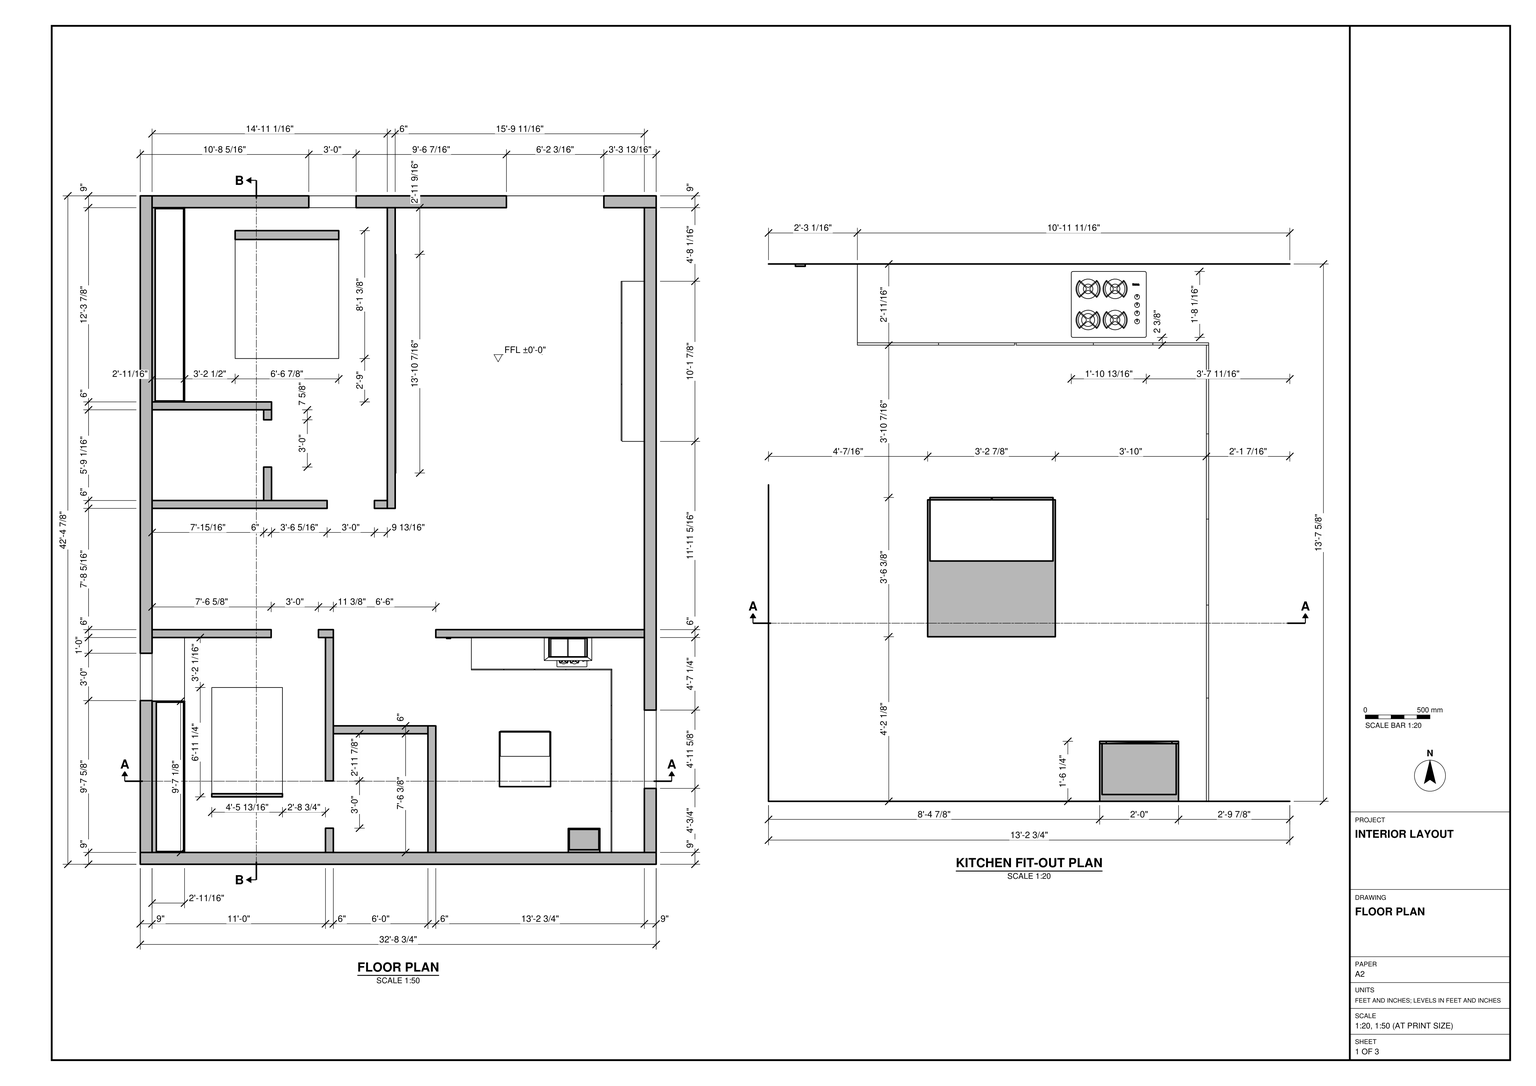
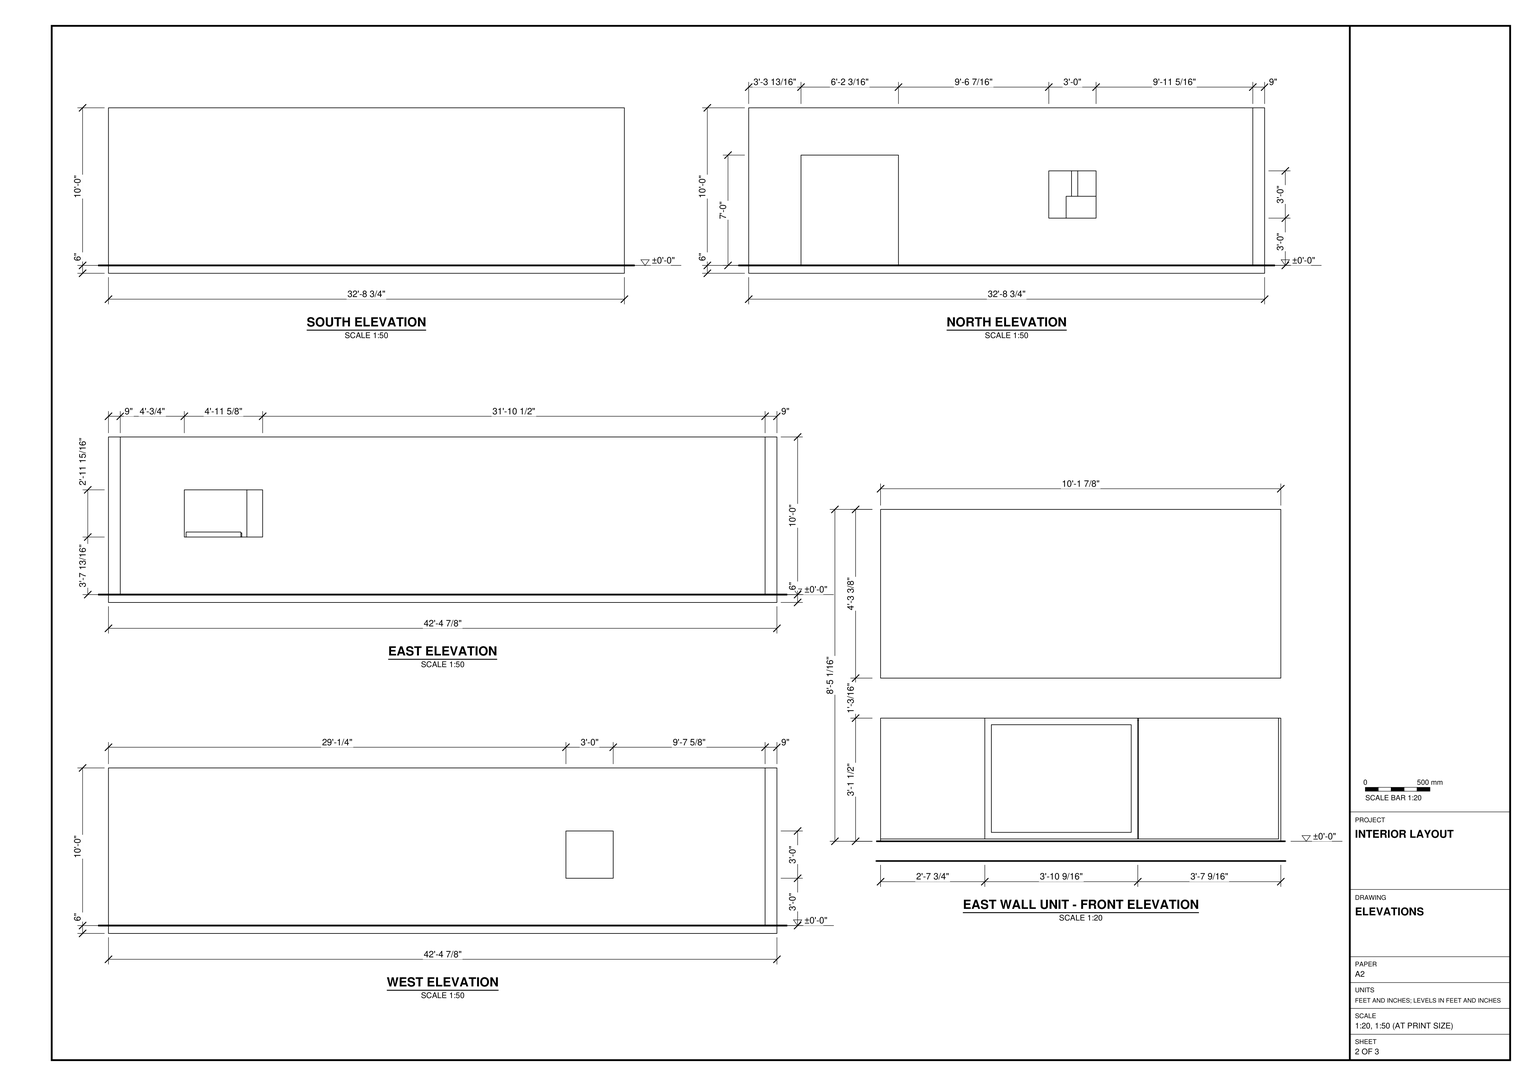
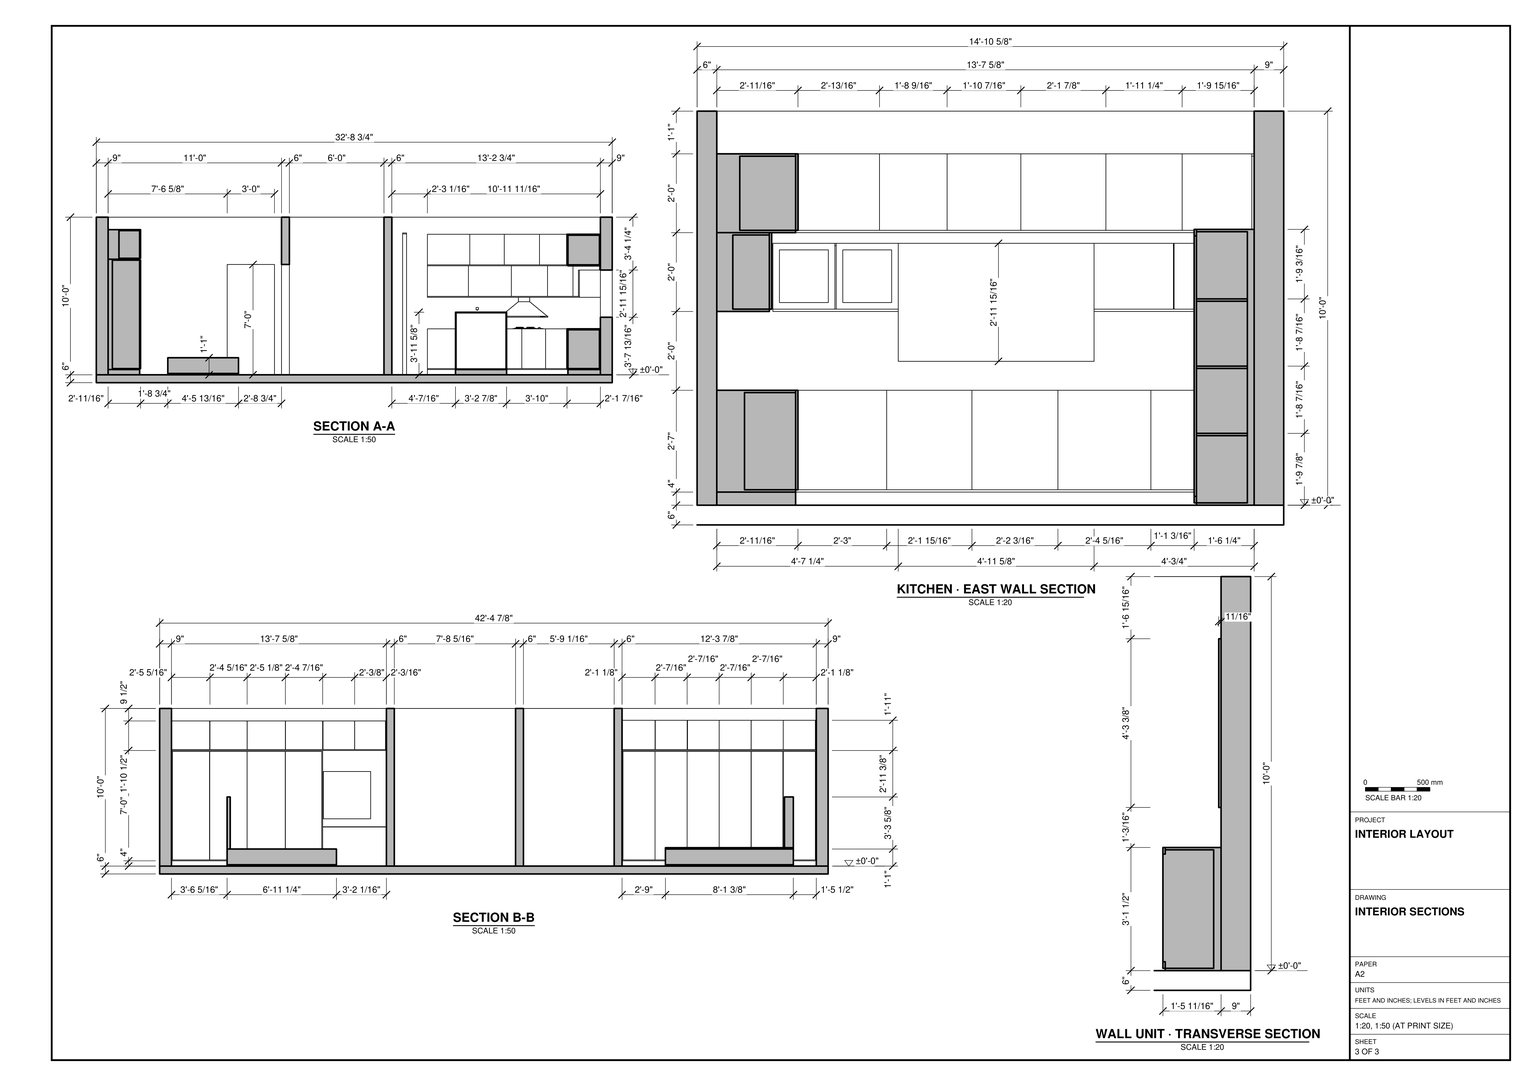
Build the interior in SketchUp from task_files/diagram_01.pdf, working in feet and inches. Set the finished floor at ±0'-0". The overall model is 32'-8 3/4" along x, 42'-4 7/8" along y and 10'-6" high, including the slab below the finished floor.

Use the floor plan to lay out the 9" perimeter walls and 6" partitions. Place the bedrooms on the west side, the kitchen in the southeast corner and the large open room to the northeast. Follow the plan for the smaller partitioned spaces and passages between rooms. Use the elevations to set the widths, heads and sills of the exterior openings.

Model each platform bed with its headboard and the adjoining west-wall storage as shown in plan and section. In the large open room, reproduce the low east-wall unit and the separate panel above it. Use the enlarged kitchen plan to locate the perimeter cabinetry, freestanding unit, cooktop and hood. Follow the kitchen section for the cabinet divisions and the way the units fit around the east-wall opening. Decor, loose items and appliances may be any suitable library components.

Keep shell elements and individual furniture and joinery pieces in separate groups or components, and use components for repeated parts. Save one SketchUp model as output_files/two_bedroom_interior_with_fitted_kitchen.skp.

# SketchUp Ruby script. Lengths in inches.
U = 1.inch
M = Sketchup.active_model
def pt(a) = Geom::Point3d.new(a.map { |v| v * U })
def face(e, loops, mat)
  f = e.add_face(loops[0].map { |a| pt(a) })
  loops[1..].each { |l| e.add_face(l.map { |a| pt(a) }).erase! }
  f.material = f.back_material = mat if mat
  f
end
# faces: each face lists its corners as indices into pts; further lists are holes
def faces(e, pts, list, mat = nil) = list.each { |f| face(e, (f[0].is_a?(Array) ? f : [f]).map { |l| l.map { |i| pts[i] } }, mat) }
# xy, xz, yz: faces in a plane at the given z, y or x. An outline is a flat list of corners, or four numbers for a rectangle; further outlines are holes
def ring(l) = l.size == 4 ? [[l[0], l[1]], [l[2], l[1]], [l[2], l[3]], [l[0], l[3]]] : l.each_slice(2).to_a
def flat(e, list, mat, &to3) = list.each { |f| face(e, (f[0].is_a?(Array) ? f : [f]).map { |l| ring(l).map { |u, v| to3.(u, v) } }, mat) }
def xy(e, z, list, mat = nil) = flat(e, list, mat) { |x, y| [x, y, z] }
def xz(e, y, list, mat = nil) = flat(e, list, mat) { |x, z| [x, y, z] }
def yz(e, x, list, mat = nil) = flat(e, list, mat) { |y, z| [x, y, z] }
def lines(e, pts, list) = list.each { |a, b| e.add_line(pt(pts[a]), pt(pts[b])) }
# prism: a flat outline (further loops are holes) pulled along v
def prism(e, loops, v, mat = nil)
  f = face(e, loops, mat); d = Geom::Vector3d.new(v.map { |x| x * U })
  f.pushpull(f.normal.samedirection?(d) ? d.length : -d.length)
end
def box(e, o, s, mat = nil) = prism(e, [[o, [o[0] + s[0], o[1], o[2]], [o[0] + s[0], o[1] + s[1], o[2]], [o[0], o[1] + s[1], o[2]]]], [0, 0, s[2]], mat)
def at(x, y, z, deg = 0) = Geom::Transformation.translation(pt([x, y, z])) * Geom::Transformation.rotation(ORIGIN, Z_AXIS, deg.degrees)
def axes(o, x, y, z) = Geom::Transformation.new([*x, 0, *y, 0, *z, 0, *pt(o).to_a, 1])
def part(name) = M.definitions.add(name)
# library, detail: a bought-in or finely detailed component or shape, given as its bounding box
def library(name, o, s) = part(name).tap { |d| box(d.entities, o, s) }
def detail(e, o, s) = box(e.add_group.entities, o, s)
def put(e, d, t, mat = nil) = e.add_instance(d, t).tap { |i| i.material = mat if mat }
def group(e, t, mat = nil) = e.add_group.tap { |g| g.transformation = t; g.material = mat if mat }.entities
root = M.entities
M.materials.add("[Translucent Glass Blue]").color = [100, 149, 237]
M.materials["[Translucent Glass Blue]"].alpha = 0.5
M.materials.add("[Translucent Glass Tinted]").color = [8, 201, 241]
M.materials["[Translucent Glass Tinted]"].alpha = 0.48
c1 = library("1-TABLE DE CUISSON CLC2",[-11.42,-10.04,0],[22.84,20.08,1.26])
c2 = library("4-PRISEELC CLC2",[-1.57,-1.58,0],[3.14,3.14,0.51])
c3 = library("1-HOTTE ASPIRANTE CLC2",[-18.13,-19.43,-0.03],[36.22,19.49,31.49])
c4 = part("Group\#47")
prism(c4.entities,[[[0,0.2,20.04],[0,19.09,20.04],[0,19.09,0],[0,0.2,0]],[[0,17.09,2],[0,17.09,18.04],[0,2.2,18.04],[0,2.2,2]]],[0.71,0,0])
c5 = part("Group\#68")
box(c5.entities,[0,0,0],[0.71,24.41,82.58])
c6 = part("Group\#85")
box(c6.entities,[0,0,0],[22.58,15.5,0.71])
box(root,[33,38.13,4.71],[0.71,28.42,82.58])
box(root,[33,9.71,4.71],[0.71,28.25,82.58])
box(root,[33,9,88.71],[0.71,29.08,21.79])
xy(root,0,[[383.75,9,392.75,499.875],[273.47,59.11,312.34,100.8],[72.23,385.02,151.1,482.39]])
xy(root,0.71,[[325.85,26.5625,349.85,27.27]])
xy(root,2.71,[[327.85,26.5625,347.85,26.5625,347.85,27.27],[327.85,26.5625,347.85,27.27,327.85,27.27]])
xy(root,4,[[273.47,59.11,312.34,100.8]])
xy(root,4.71,[[274.17,82.18,311.63,100.8]])
xy(root,43.8125,[[383.75,57.75,392.75,117.375]])
xy(root,46.92,[[274.17,82.18,311.63,100.8]])
xy(root,47.625,[[273.47,59.11,312.34,100.8]])
xy(root,79.75,[[383.75,57.75,392.75,117.375]])
xy(root,82,[[327.85,26.5625,327.85,27.27,347.85,27.27],[327.85,26.5625,347.85,27.27,347.85,26.5625]])
xy(root,84,[[325.85,26.5625,349.85,27.27]])
xy(root,120,[[383.75,9,392.75,499.875]])
xz(root,9,[[383.75,0,392.75,120]])
xz(root,26.5625,[[[325.85,0.71,349.85,84],[327.85,2.71,347.85,82]],[327.85,2.71,347.85,82]])
xz(root,27.27,[[[325.85,0.71,349.85,84],[327.85,2.71,347.85,82]]])
xz(root,27.27,[[327.85,2.71,347.85,82]],"[Translucent Glass Tinted]")
xz(root,57.75,[[383.75,43.8125,392.75,79.75]])
xz(root,59.11,[[273.47,0,312.34,4],[273.47,4,312.34,47.625]])
xz(root,82.18,[[274.17,4.71,311.63,46.92]])
xz(root,100.8,[[273.47,0,312.34,4],[[273.47,4,312.34,47.625],[274.17,4.71,311.63,46.92]]])
xz(root,117.375,[[383.75,43.8125,392.75,79.75]])
xz(root,499.875,[[383.75,0,392.75,120]])
yz(root,273.47,[[59.11,0,100.8,4],[59.11,4,100.8,47.625]])
yz(root,274.17,[[82.18,4.71,100.8,46.92]])
yz(root,311.63,[[82.18,4.71,100.8,46.92]])
yz(root,312.34,[[59.11,0,100.8,4],[59.11,4,100.8,47.625]])
yz(root,325.85,[[26.5625,0.71,27.27,84]])
yz(root,327.85,[[26.5625,2.71,27.27,82]])
yz(root,347.85,[[26.5625,2.71,27.27,82]])
yz(root,349.85,[[26.5625,0.71,27.27,84]])
yz(root,366.04,[[367.49,2.71,410.07,35.5]],"[Translucent Glass Blue]")
yz(root,383.75,[[9,0,9,59,57.75,59,57.75,43.8125,117.375,43.8125,117.375,59,155.55,59,155.55,79.75,9,79.75,9,120,499.875,120,499.875,0]])
yz(root,392.75,[[[9,0,499.875,120],[57.75,43.8125,117.375,79.75]]])
p = [[327.85,26.5625,2.71],[347.85,27.27,2.71],[347.85,27.27,82],[327.85,26.5625,82],[33,37.96,87.29],[33,38.13,87.29]]
faces(root,p,[[0,1,2,3]])
lines(root,p,[[4,5]])
put(root,c1,at(328.62,160.3125,35))
put(root,c2,axes([289.98,172.625,50.39],[1,0,0],[0,0,1],[0,-1,0]))
put(root,c3,at(325.66,172.57,43.88))
g1 = group(root,at(0,0,0))
box(g1,[0,0,0],[392.75,9,120])
g2 = group(root,at(0,9,0))
prism(g2,[[[0,499.875,0],[0,0,0],[0,0,120],[0,499.875,120]],[[0,151.625,72],[0,115.625,72],[0,115.625,36],[0,151.625,36]]],[9,0,0])
g3 = group(root,at(141,9,0))
prism(g3,[[[6,0,0],[6,18.47,0],[6,18.47,84],[6,54.47,84],[6,54.47,0],[6,163.625,0],[6,163.625,120],[6,0,120]]],[-6,0,0])
g4 = group(root,at(9,172.625,0))
prism(g4,[[[0,0,0],[90.65,0,0],[90.65,0,84],[126.65,0,84],[126.65,0,0],[138,0,0],[138,0,120],[0,0,120]]],[0,6,0])
g5 = group(root,at(219,9,0))
box(g5,[0,0,0],[6,96.375,120])
g6 = group(root,at(147,99.375,0))
box(g6,[0,0,0],[72,6,120])
g7 = group(root,at(225,172.625,0))
box(g7,[0,0,0],[158.75,6,120])
g8 = group(root,at(9,499.875,0))
prism(g8,[[[343.9375,0,0],[383.75,0,0],[383.75,0,120],[0,0,120],[0,0,0],[269.75,0,0],[269.75,0,84],[343.9375,0,84]],[[155.3125,0,72],[155.3125,0,36],[119.3125,0,36],[119.3125,0,72]]],[0,9,0])
g9 = group(root,at(188.0625,270.9375,0))
box(g9,[0,0,0],[6,228.9375,120])
g10 = group(root,at(9,270.9375,0))
prism(g10,[[[133.25,6,0],[0,6,0],[0,6,120],[179.0625,6,120],[179.0625,6,0],[169.25,6,0],[169.25,6,84],[133.25,6,84]]],[0,-6,0])
g11 = group(root,at(0,0,-6))
box(g11,[0,0,0],[392.75,508.875,6])
g12 = group(root,at(252.0625,148.625,0))
prism(g12,[[[131.6875,24,0],[131.6875,-145,0],[106.98,-145,0],[106.98,0,0],[0,0,0],[0,24,0]]],[0,0,4])
g13 = group(root,at(252.0625,148.625,4))
xy(g13,0,[[106.98,-139.625,106.98,0,0,0,0,24,131.6875,24,131.6875,-139.625]])
xy(g13,0.71,[[106.98,-139.625,130.98,-139.625,130.98,15.5625,0.71,15.5625,0.71,0,106.98,0]])
xy(g13,30.29,[[106.98,-139.625,106.98,0,0.71,0,0.71,15.5625,130.98,15.5625,130.98,-139.625]])
xy(g13,31,[[106.98,-139.625,131.6875,-139.625,131.6875,24,0,24,0,0,106.98,0]])
xz(g13,-139.625,[[106.98,0,131.6875,0,131.6875,31,106.98,31,106.98,30.29,130.98,30.29,130.98,0.71,106.98,0.71]])
xz(g13,0,[[0,0,106.98,0,106.98,0.71,0.71,0.71,0.71,30.29,106.98,30.29,106.98,31,0,31]])
xz(g13,15.5625,[[0.71,0.71,130.98,30.29]])
xz(g13,24,[[0,0,131.6875,31]])
yz(g13,0,[[0,0,24,31]])
yz(g13,0.71,[[0,0.71,15.5625,30.29]])
yz(g13,106.98,[[-139.625,0,0,0.71],[-139.625,30.29,0,31]])
yz(g13,130.98,[[-139.625,0.71,15.5625,30.29]])
yz(g13,131.6875,[[-139.625,0,24,31]])
g14 = group(root,at(359.04,9,4.71))
box(g14,[0,0,0],[24,0.71,29.5625])
g15 = group(root,at(252.0625,147.92,4.71))
box(g15,[0,0,0],[24.71,0.71,30.29])
g16 = group(root,at(276.77,147.92,4.71))
box(g16,[0,0,0],[23.15,0.71,30.29])
g17 = group(root,at(300.4,147.92,4.71))
box(g17,[0,0,0],[23.53,0.71,30.29])
g18 = group(root,at(323.92,147.92,4.71))
box(g18,[0,0,0],[18.12,0.71,30.29])
g19 = group(root,at(342.04,147.92,4.71))
box(g19,[0,0,0],[17,0.71,30.29])
g20 = group(root,at(358.33,120.89,4.71))
box(g20,[0,0,0],[0.71,27.03,30.29])
g21 = group(root,at(358.33,94.9375,4.71))
box(g21,[0,0,0],[0.71,25.95,30.29])
g22 = group(root,at(358.33,68.75,4.71))
box(g22,[0,0,0],[0.71,26.18,30.29])
g23 = group(root,at(358.33,40.44,4.71))
box(g23,[0,0,0],[0.71,28.31,30.29])
g24 = group(root,at(358.33,9.71,4.71))
box(g24,[0,-0.71,0],[0.71,31.44,30.29])
g25 = group(root,at(252.0625,172.625,59))
xy(g25,0,[[0,-16,131.6875,0]])
xy(g25,0.71,[[0.71,-16,130.98,-4.875]])
xy(g25,23.29,[[0.71,-16,130.98,-4.875]])
xy(g25,24,[[0,-16,131.6875,0]])
xz(g25,-16,[[[0,0,131.6875,24],[0.71,0.71,130.98,23.29]]])
xz(g25,-4.875,[[0.71,0.71,130.98,23.29]])
xz(g25,0,[[0,0,131.6875,24]])
yz(g25,0,[[-16,0,0,24]])
yz(g25,0.71,[[-16,0.71,-4.875,23.29]])
yz(g25,130.98,[[-16,0.71,-4.875,23.29]])
yz(g25,131.6875,[[-16,0,0,24]])
g26 = group(root,at(252.0625,155.92,59.71))
box(g26,[0,0,0],[31.24,0.71,23.29])
g27 = group(root,at(283.3,155.92,59.71))
box(g27,[0,0,0],[32.65,0.71,23.29])
g28 = group(root,at(315.96,155.92,59.71))
box(g28,[0,0,0],[27.54,0.71,23.29])
g29 = group(root,at(343.49,155.92,59.71))
box(g29,[0,0,0],[19.39,0.71,23.29])
g30 = group(root,at(362.88,155.92,59.71))
box(g30,[0,0,0],[20.16,0.71,23.29])
g31 = group(root,at(252.0625,172.625,83))
xy(g31,0,[[106.98,-163.625,106.98,-24,0,-24,0,0,131.6875,0,131.6875,-163.625]])
xy(g31,0.71,[[106.98,-163.625,130.98,-163.625,130.98,-7,0.71,-7,0.71,-24,106.98,-24]])
xy(g31,23.29,[[106.98,-163.625,106.98,-24,0.71,-24,0.71,-7,130.98,-7,130.98,-163.625]])
xy(g31,24,[[106.98,-163.625,131.6875,-163.625,131.6875,0,0,0,0,-24,106.98,-24]])
xz(g31,-163.625,[[106.98,0,131.6875,0,131.6875,24,106.98,24,106.98,23.29,130.98,23.29,130.98,0.71,106.98,0.71]])
xz(g31,-24,[[0,0,106.98,0,106.98,0.71,0.71,0.71,0.71,23.29,106.98,23.29,106.98,24,0,24]])
xz(g31,-7,[[0.71,0.71,130.98,23.29]])
xz(g31,0,[[0,0,131.6875,24]])
yz(g31,0,[[-24,0,0,24]])
yz(g31,0.71,[[-24,0.71,-7,23.29]])
yz(g31,106.98,[[-163.625,0,-24,0.71],[-163.625,23.29,-24,24]])
yz(g31,130.98,[[-163.625,0.71,-7,23.29]])
yz(g31,131.6875,[[-163.625,0,0,24]])
g32 = group(root,at(359.04,9,83.71))
box(g32,[0,0,0],[24,0.71,22.58])
g33 = group(root,at(252.0625,147.92,83.71))
box(g33,[0,0,0],[32.26,0.71,23.29])
g34 = group(root,at(284.32,147.92,83.71))
box(g34,[0,0,0],[26.24,0.71,23.29])
g35 = group(root,at(310.57,147.92,83.71))
box(g35,[0,0,0],[26.82,0.71,23.29])
g36 = group(root,at(337.39,147.92,83.71))
box(g36,[0,0,0],[21.65,0.71,23.29])
g37 = group(root,at(358.33,123.08,83.71))
box(g37,[0,0,0],[0.71,24.65,23.29])
g38 = group(root,at(358.33,102.49,83.71))
box(g38,[0,0,0],[0.71,20.59,23.29])
g39 = group(root,at(358.33,80.04,83.71))
box(g39,[0,0,0],[0.71,22.45,23.29])
g40 = group(root,at(358.33,54.15,83.71))
box(g40,[0,0,0],[0.71,25.89,23.29])
g41 = group(root,at(358.33,30.92,83.71))
box(g41,[0,0,0],[0.71,23.23,23.29])
g42 = group(root,at(358.33,9.71,83.71))
box(g42,[0,0,0],[0.71,21.21,23.29])
g43 = group(root,at(292.9,100.8,4.71))
box(g43,[0.2,0,0],[18.53,0.71,42.21])
g44 = group(root,at(273.97,100.8,4.71))
box(g44,[0.2,0,0],[18.72,0.71,42.21])
g45 = group(root,at(383.75,117.375,59))
xy(g45,0,[[-16,0,0,38.17]])
xy(g45,0.71,[[-16,0.71,-3.875,37.46]])
xy(g45,20.04,[[-16,0.71,-3.875,37.46]])
xy(g45,20.75,[[-16,0,0,38.17]])
xz(g45,0,[[-16,0,0,20.75]])
xz(g45,0.71,[[-16,0.71,-3.875,20.04]])
xz(g45,37.46,[[-16,0.71,-3.875,20.04]])
xz(g45,38.17,[[-16,0,0,20.75]])
yz(g45,-16,[[[0,0,38.17,20.75],[0.71,0.71,37.46,20.04]]])
yz(g45,-3.875,[[0.71,0.71,37.46,20.04]])
yz(g45,0,[[0,0,38.17,20.75]])
put(root,c4,at(367.04,136.46,59.71))
put(root,c4,at(367.04,117.18,59.71))
g46 = group(root,at(383.75,9,59))
xy(g46,0,[[-16,0,0,48.75]])
xy(g46,0.71,[[-16,0.71,-3.75,48.04]])
xy(g46,20.04,[[-16,0.71,-3.75,48.04]])
xy(g46,20.75,[[-16,0,0,48.75]])
xz(g46,0,[[-16,0,0,20.75]])
xz(g46,0.71,[[-16,0.71,-3.75,20.04]])
xz(g46,48.04,[[-16,0.71,-3.75,20.04]])
xz(g46,48.75,[[-16,0,0,20.75]])
yz(g46,-16,[[[0,0,48.75,20.75],[0.71,0.71,48.04,20.04]]])
yz(g46,-3.75,[[0.71,0.71,48.04,20.04]])
yz(g46,0,[[0,0,48.75,20.75]])
g47 = group(root,at(367.04,33.375,59.71))
box(g47,[0,0.2,0],[0.71,24.18,20.04])
g48 = group(root,at(367.04,9.71,59.71))
box(g48,[0,0,0],[0.71,23.67,20.04])
g49 = group(root,at(9,9,0))
box(g49,[0,0,0],[24,115.11,4])
g50 = group(root,at(9,9,4))
xy(g50,0,[[0,0,24,115.11]])
xy(g50,0.71,[[3.25,0.71,24,114.4]])
xy(g50,83.29,[[3.25,0.71,24,114.4]])
xy(g50,84,[[0,0,24,115.11]])
xz(g50,0,[[0,0,24,84]])
xz(g50,0.71,[[3.25,0.71,24,83.29]])
xz(g50,114.4,[[3.25,0.71,24,83.29]])
xz(g50,115.11,[[0,0,24,84]])
yz(g50,0,[[0,0,115.11,84]])
yz(g50,3.25,[[0.71,0.71,114.4,83.29]])
yz(g50,24,[[[0,0,115.11,84],[0.71,0.71,114.4,83.29]]])
g51 = group(root,at(33,95.72,4.71))
box(g51,[0,0,0],[0.71,27.68,82.58])
g52 = group(root,at(33,66.58,4.71))
box(g52,[0,0,0],[0.71,29.05,82.58])
g53 = group(root,at(9,9,88))
xy(g53,0,[[0,0,24,163.625]])
xy(g53,0.71,[[8.25,0.71,24,162.92]])
xy(g53,21.79,[[8.25,0.71,24,162.92]])
xy(g53,22.5,[[0,0,24,163.625]])
xz(g53,0,[[0,0,24,22.5]])
xz(g53,0.71,[[8.25,0.71,24,21.79]])
xz(g53,162.92,[[8.25,0.71,24,21.79]])
xz(g53,163.625,[[0,0,24,22.5]])
yz(g53,0,[[0,0,163.625,22.5]])
yz(g53,8.25,[[0.71,0.71,162.92,21.79]])
yz(g53,24,[[[0,0,163.625,22.5],[0.71,0.71,162.92,21.79]]])
g54 = group(root,at(33,38.28,88.71))
box(g54,[0,0,0],[0.71,28.3,21.79])
g55 = group(root,at(33,66.65,88.71))
box(g55,[0,0,0],[0.71,29.05,21.79])
g56 = group(root,at(33,95.81,88.71))
box(g56,[0,0,0],[0.71,28.27,21.79])
g57 = group(root,at(33,124.37,88.71))
box(g57,[0,0,0],[0.71,24.04,21.79])
g58 = group(root,at(33,148.47,88.71))
box(g58,[0,0,0],[0.71,23.45,21.79])
g59 = group(root,at(9,124.43,29.74))
box(g59,[0,0,0],[24.71,48.2,0.2])
g60 = group(root,at(9,346,0))
box(g60,[0,0,0],[90.9375,6,120])
g61 = group(root,at(93.9375,276.9375,0))
prism(g61,[[[0,69.0625,0],[0,61.4375,0],[0,61.4375,84],[0,25.4375,84],[0,25.4375,0],[0,0,0],[0,0,120],[0,69.0625,120]]],[6,0,0])
g62 = group(root,at(9,352,0))
box(g62,[0,0,0],[24,147.875,4])
g63 = group(root,at(9,352,4))
xy(g63,0,[[0,0,24,147.875]])
xy(g63,0.71,[[2.375,0.71,24,147.17]])
xy(g63,83.29,[[2.375,0.71,24,147.17]])
xy(g63,84,[[0,0,24,147.875]])
xz(g63,0,[[0,0,24,84]])
xz(g63,0.71,[[2.375,0.71,24,83.29]])
xz(g63,147.17,[[2.375,0.71,24,83.29]])
xz(g63,147.875,[[0,0,24,84]])
yz(g63,0,[[0,0,147.875,84]])
yz(g63,2.375,[[0.71,0.71,147.17,83.29]])
yz(g63,24,[[[0,0,147.875,84],[0.71,0.71,147.17,83.29]]])
g64 = group(root,at(33,474.76,4.71))
box(g64,[0,0,0],[0.71,24.41,82.58])
g65 = group(root,at(33,450.35,4.71))
box(g65,[0,0,0],[0.71,24.1,82.58])
g66 = group(root,at(33,425.9375,4.71))
box(g66,[0,0,0],[0.71,24.27,82.58])
put(root,c5,at(33,401.53,4.71))
put(root,c5,at(33,377.12,4.71))
put(root,c5,at(33,352.71,4.71))
g67 = group(root,at(9,352,88))
xy(g67,0,[[0,0,24,147.875]])
xy(g67,0.71,[[8.6875,0.71,24,147.17]])
xy(g67,22.29,[[8.6875,0.71,24,147.17]])
xy(g67,23,[[0,0,24,147.875]])
xz(g67,0,[[0,0,24,23]])
xz(g67,0.71,[[8.6875,0.71,24,22.29]])
xz(g67,147.17,[[8.6875,0.71,24,22.29]])
xz(g67,147.875,[[0,0,24,23]])
yz(g67,0,[[0,0,147.875,23]])
yz(g67,8.6875,[[0.71,0.71,147.17,22.29]])
yz(g67,24,[[[0,0,147.875,23],[0.71,0.71,147.17,22.29]]])
g68 = group(root,at(33,352,88.71))
box(g68,[0,0,0],[0.71,25.13,22.29])
g69 = group(root,at(33,377.3,88.71))
box(g69,[0,0,0],[0.71,24.27,22.29])
g70 = group(root,at(33,401.82,88.71))
box(g70,[0,0,0],[0.71,24.12,22.29])
g71 = group(root,at(33,425.9375,88.71))
box(g71,[0,0,0],[0.71,24.32,22.29])
g72 = group(root,at(33,450.31,88.71))
box(g72,[0,0,0],[0.71,24.39,22.29])
g73 = group(root,at(33,474.69,88.71))
box(g73,[0,0,0],[0.71,24.47,22.29])
g74 = group(root,at(383.75,443.8125,0))
xy(g74,0,[[-17,-121.875,0,0]])
xy(g74,0.71,[[-17,-121.17,-2.25,-0.71]])
xy(g74,36.79,[[-17,-121.17,-2.25,-0.71]])
xy(g74,37.5,[[-17,-121.875,0,0]])
xz(g74,-121.875,[[-17,0,0,37.5]])
xz(g74,-121.17,[[-17,0.71,-2.25,36.79]])
xz(g74,-0.71,[[-17,0.71,-2.25,36.79]])
xz(g74,0,[[-17,0,0,37.5]])
yz(g74,-17,[[[-121.875,0,0,37.5],[-121.17,0.71,-0.71,36.79]]])
yz(g74,-2.25,[[-121.17,0.71,-0.71,36.79]])
yz(g74,0,[[-121.875,0,0,37.5]])
g75 = group(root,at(366.04,412.07,0.71))
box(g75,[0,0,0],[0.71,31.74,36.79])
g76 = group(root,at(366.04,365.49,0.71))
prism(g76,[[[0.71,46.58,0],[0.71,46.58,36.79],[0.71,0,36.79],[0.71,0,0]],[[0.71,2,34.79],[0.71,44.58,34.79],[0.71,44.58,2],[0.71,2,2]]],[-0.71,0,0])
g77 = group(root,at(366.04,322.65,0.71))
box(g77,[0,0,0],[0.71,42.67,36.79])
g78 = group(root,at(383.75,443.8125,49.6875))
box(g78,[-0.71,-121.875,0],[0.71,121.875,51.375])
g79 = group(root,at(54.44,51.33,0))
box(g79,[0,0,0],[53.8125,83.25,1])
g80 = group(root,at(54.44,51.33,1))
box(g80,[0,0,0],[53.8125,83.25,12])
g81 = group(root,at(54.44,51.33,13))
box(g81,[0,0,0],[53.8125,2.375,39.625])
g82 = group(root,at(325.85,9,0))
xy(g82,0,[[0,0,24,17.5625]])
xy(g82,0.71,[[0.71,2.0625,23.29,17.5625]])
xy(g82,83.29,[[0.71,2.0625,23.29,17.5625]])
xy(g82,84,[[0,0,24,17.5625]])
xz(g82,0,[[0,0,24,84]])
xz(g82,2.0625,[[0.71,0.71,23.29,83.29]])
xz(g82,17.5625,[[[0,0,24,84],[0.71,0.71,23.29,83.29]]])
yz(g82,0,[[0,0,17.5625,84]])
yz(g82,0.71,[[2.0625,0.71,17.5625,83.29]])
yz(g82,23.29,[[2.0625,0.71,17.5625,83.29]])
yz(g82,24,[[0,0,17.5625,84]])
put(root,c6,at(326.5625,11.0625,21.18))
put(root,c6,at(326.5625,11.0625,41.65))
put(root,c6,at(326.5625,11.0625,62.11))
g83 = group(root,at(72.23,385.02,0))
xy(g83,0,[[0,0,78.875,97.375]])
xz(g83,0,[[0,0,78.875,1]])
xz(g83,97.375,[[0,0,78.875,1]])
yz(g83,0,[[0,0,97.375,1]])
yz(g83,78.875,[[0,0,97.375,1]])
g84 = group(g83,at(0,0,1))
box(g84,[0,0,0],[78.875,97.375,12])
g85 = group(root,at(72.23,385.02,13))
box(g85,[0,0,0],[78.875,97.375,1])
g86 = group(root,at(72.23,475.64,14))
box(g86,[0,0,0],[78.875,6.75,38.625])
g87 = group(root,at(194.0625,297.875,33.03))
box(g87,[0,0,0],[0.3125,166.4375,64.5625])
g88 = group(root,at(233.2,172.625,0))
box(g88,[0,-0.71,0],[2.99,0.71,108])
g89 = group(root,at(233.2,171.92,107.25))
box(g89,[0,-46.75,0],[2.99,46.75,0.75])
